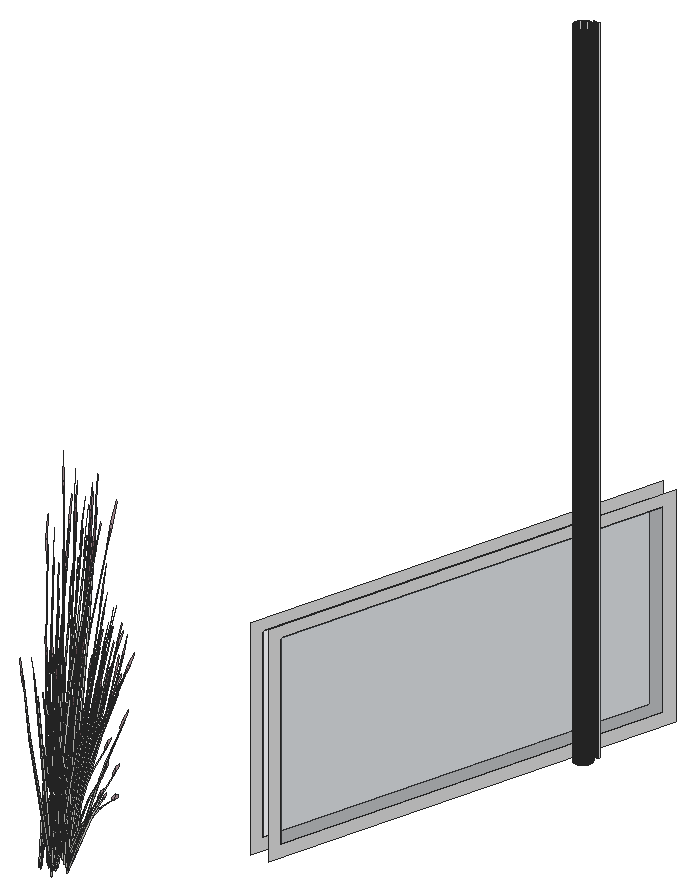
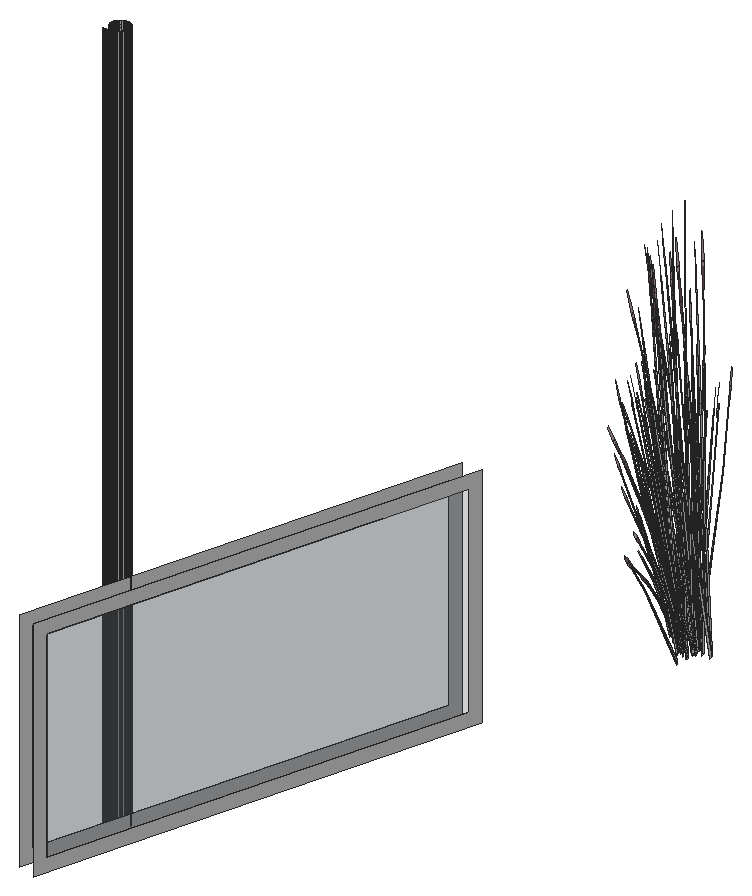
# SketchUp Ruby script. Lengths in inches.
U = 1.inch
M = Sketchup.active_model
def pt(a) = Geom::Point3d.new(a.map { |v| v * U })
def face(e, loops, mat)
  f = e.add_face(loops[0].map { |a| pt(a) })
  loops[1..].each { |l| e.add_face(l.map { |a| pt(a) }).erase! }
  f.material = f.back_material = mat if mat
  f
end
# faces: each face lists its corners as indices into pts; further lists are holes
def faces(e, pts, list, mat = nil) = list.each { |f| face(e, (f[0].is_a?(Array) ? f : [f]).map { |l| l.map { |i| pts[i] } }, mat) }
# xy, xz, yz: faces in a plane at the given z, y or x. An outline is a flat list of corners, or four numbers for a rectangle; further outlines are holes
def ring(l) = l.size == 4 ? [[l[0], l[1]], [l[2], l[1]], [l[2], l[3]], [l[0], l[3]]] : l.each_slice(2).to_a
def flat(e, list, mat, &to3) = list.each { |f| face(e, (f[0].is_a?(Array) ? f : [f]).map { |l| ring(l).map { |u, v| to3.(u, v) } }, mat) }
def xy(e, z, list, mat = nil) = flat(e, list, mat) { |x, y| [x, y, z] }
def xz(e, y, list, mat = nil) = flat(e, list, mat) { |x, z| [x, y, z] }
def yz(e, x, list, mat = nil) = flat(e, list, mat) { |y, z| [x, y, z] }
def lines(e, pts, list) = list.each { |a, b| e.add_line(pt(pts[a]), pt(pts[b])) }
# prism: a flat outline (further loops are holes) pulled along v
def prism(e, loops, v, mat = nil)
  f = face(e, loops, mat); d = Geom::Vector3d.new(v.map { |x| x * U })
  f.pushpull(f.normal.samedirection?(d) ? d.length : -d.length)
end
def box(e, o, s, mat = nil) = prism(e, [[o, [o[0] + s[0], o[1], o[2]], [o[0] + s[0], o[1] + s[1], o[2]], [o[0], o[1] + s[1], o[2]]]], [0, 0, s[2]], mat)
def at(x, y, z, deg = 0) = Geom::Transformation.translation(pt([x, y, z])) * Geom::Transformation.rotation(ORIGIN, Z_AXIS, deg.degrees)
def axes(o, x, y, z) = Geom::Transformation.new([*x, 0, *y, 0, *z, 0, *pt(o).to_a, 1])
def part(name) = M.definitions.add(name)
# library, detail: a bought-in or finely detailed component or shape, given as its bounding box
def library(name, o, s) = part(name).tap { |d| box(d.entities, o, s) }
def detail(e, o, s) = box(e.add_group.entities, o, s)
def put(e, d, t, mat = nil) = e.add_instance(d, t).tap { |i| i.material = mat if mat }
def group(e, t, mat = nil) = e.add_group.tap { |g| g.transformation = t; g.material = mat if mat }.entities
root = M.entities
M.materials.add("Glass_Basic_01").color = [105, 113, 122]
M.materials["Glass_Basic_01"].alpha = 0.25
M.materials.add("LightPink_Translucent").color = [144, 107, 117]
M.materials["LightPink_Translucent"].alpha = 0.75
M.materials.add("M01_Silver_Fog").color = [224, 224, 224]
c1 = part("blade")
p = [[2.15,0.21,22],[0,0.17,0],[0.09,0.45,0],[2.18,0.31,22],[2.29,0.31,22],[0.38,0.45,0],
  [2.48,0.24,33],[2.49,0.24,33],[2.48,0.22,33]]
faces(c1.entities,p,[[0,1,2,3],[4,5,2,3],[6,3,4,7],[8,0,3,6]])
c2 = part("seeds")
p = [[0.3,-0.1,1.38],[-0.01,-0.03,1.59],[-0.01,-0.03,0.03],[0.14,-0.07,-0.07],[0.29,-0.03,3],[0.15,0.01,3.11]]
faces(c2.entities,p,[[0,1,2,3],[1,0,4,5]],"LightPink_Translucent")
c3 = part("blade with seeds")
put(c3.entities,c1,at(0,0,0))
put(c3.entities,c2,axes([2.4,0.25,30.99],[1.5799,-0.05474,1.17369],[-0.12525,1.92788,0.29478],[-0.07173,-0.02425,1.56792]))
xz(root,421.6,[[358.82,270,358.91,384],[358.91,270,359,384]],"M01_Silver_Fog")
xz(root,421.95,[[359.74,270,359.83,384],[359.83,270,359.92,384]],"M01_Silver_Fog")
yz(root,357.51,[[420.11,270,420.2,384],[420.2,270,420.29,384]],"M01_Silver_Fog")
yz(root,360.31,[[420.11,270,420.2,384],[420.2,270,420.29,384]],"M01_Silver_Fog")
p = [[359.17,437.01,270],[340.07,371.78,270],[340.07,371.78,306],[359.17,437.01,306],[340.64,373.7,272],[358.6,435.09,272],
  [358.6,435.09,304],[340.64,373.7,304],[362.06,436.22,306],[343.2,371.78,306],[343.2,371.78,270],[362.06,436.22,270],
  [343.76,373.7,304],[361.5,434.3,304],[361.5,434.3,272],[343.76,373.7,272],[358.48,418.87,270],[358.5625,418.85,270],
  [358.5625,418.85,384],[358.48,418.87,384],[358.65,418.83,270],[358.73,418.8125,270],[358.73,418.8125,384],[358.65,418.83,384],
  [358.82,418.81,270],[358.82,418.81,384],[358.91,418.8,270],[358.91,418.8,384],[359,418.81,270],[359,418.81,384],
  [359.09,418.8125,270],[359.09,418.8125,384],[359.17,418.83,270],[359.17,418.83,384],[359.26,418.85,270],[359.26,418.85,384],
  [359.34,418.87,270],[359.34,418.87,384],[358.24,418.98,270],[358.3125,418.9375,270],[358.3125,418.9375,384],[358.24,418.98,384],
  [358.39,418.9,270],[358.39,418.9,384],[359.43,418.9,270],[359.43,418.9,384],[359.51,418.9375,270],[359.51,418.9375,384],
  [359.58,418.98,270],[359.58,418.98,384],[358.09,419.07,270],[358.16,419.02,270],[358.16,419.02,384],[358.09,419.07,384],
  [359.66,419.02,270],[359.66,419.02,384],[359.73,419.07,270],[359.73,419.07,384],[358.02,419.125,270],[358.02,419.125,384],
  [357.95,419.18,270],[357.95,419.18,384],[359.8,419.125,270],[359.8,419.125,384],[359.87,419.18,270],[359.87,419.18,384],
  [357.83,419.31,270],[357.89,419.24,270],[357.89,419.24,384],[357.83,419.31,384],[359.93,419.24,270],[359.93,419.24,384],
  [359.99,419.31,270],[359.99,419.31,384],[357.78,419.38,270],[357.78,419.38,384],[360.04,419.38,270],[360.04,419.38,384],
  [357.73,419.45,270],[357.73,419.45,384],[360.09,419.45,270],[360.09,419.45,384],[357.64,419.61,270],[357.68,419.53,270],
  [357.68,419.53,384],[357.64,419.61,384],[360.14,419.53,270],[360.14,419.53,384],[360.18,419.61,270],[360.18,419.61,384],
  [357.61,419.6875,270],[357.61,419.6875,384],[360.21,419.6875,270],[360.21,419.6875,384],[357.58,419.77,270],[357.58,419.77,384],
  [360.24,419.77,270],[360.24,419.77,384],[357.55,419.85,270],[357.55,419.85,384],[360.27,419.85,270],[360.27,419.85,384],
  [357.54,419.94,270],[357.54,419.94,384],[357.52,420.03,270],[357.52,420.03,384],[360.29,419.94,270],[360.29,419.94,384],
  [360.3,420.03,270],[360.3,420.03,384],[357.51,420.11,270],[357.51,420.11,384],[360.31,420.11,270],[360.31,420.11,384],
  [357.52,420.38,270],[357.51,420.29,270],[357.51,420.29,384],[357.52,420.38,384],[360.31,420.29,270],[360.3,420.38,270],
  [360.3,420.38,384],[360.31,420.29,384],[357.54,420.46,270],[357.54,420.46,384],[360.29,420.46,270],[360.29,420.46,384],
  [357.55,420.55,270],[357.55,420.55,384],[360.27,420.55,270],[360.27,420.55,384],[357.58,420.64,270],[357.58,420.64,384],
  [357.61,420.72,270],[357.61,420.72,384],[360.24,420.64,270],[360.24,420.64,384],[360.21,420.72,270],[360.21,420.72,384],
  [357.64,420.8,270],[357.64,420.8,384],[360.18,420.8,270],[360.18,420.8,384],[357.68,420.88,270],[357.68,420.88,384],
  [360.14,420.88,270],[360.14,420.88,384],[357.73,420.95,270],[357.73,420.95,384],[360.09,420.95,270],[360.09,420.95,384],
  [357.78,421.03,270],[357.78,421.03,384],[357.83,421.09,270],[357.83,421.09,384],[360.04,421.03,270],[360.04,421.03,384],
  [359.99,421.09,270],[359.99,421.09,384],[357.89,421.16,270],[357.89,421.16,384],[359.93,421.16,270],[359.93,421.16,384],
  [357.95,421.22,270],[357.95,421.22,384],[358.02,421.28,270],[358.02,421.28,384],[359.87,421.22,270],[359.8,421.28,270],
  [359.8,421.28,384],[359.87,421.22,384],[358.09,421.34,270],[358.09,421.34,384],[358.16,421.38,270],[358.16,421.38,384],
  [359.73,421.34,270],[359.73,421.34,384],[359.66,421.38,270],[359.66,421.38,384],[358.24,421.43,270],[358.24,421.43,384],
  [358.3125,421.47,270],[358.3125,421.47,384],[359.58,421.43,270],[359.51,421.47,270],[359.51,421.47,384],[359.58,421.43,384],
  [358.39,421.5,270],[358.39,421.5,384],[358.48,421.53,270],[358.48,421.53,384],[358.5625,421.56,270],[358.5625,421.56,384],
  [359.43,421.5,270],[359.34,421.53,270],[359.34,421.53,384],[359.43,421.5,384],[359.26,421.56,270],[359.26,421.56,384],
  [358.65,421.58,270],[358.65,421.58,384],[358.73,421.59,270],[358.73,421.59,384],[358.82,421.6,270],[358.82,421.6,384],
  [359.09,421.59,270],[359,421.6,270],[359,421.6,384],[359.09,421.59,384],[359.17,421.58,270],[359.17,421.58,384],
  [359.66,421.96,270],[359.74,421.95,270],[359.74,421.95,384],[359.66,421.96,384],[359.92,421.95,270],[360.01,421.96,270],
  [360.01,421.96,384],[359.92,421.95,384],[359.32,422.05,270],[359.4,422.02,270],[359.4,422.02,384],[359.32,422.05,384],
  [359.48,421.99,270],[359.48,421.99,384],[359.57,421.97,270],[359.57,421.97,384],[360.09,421.97,270],[360.09,421.97,384],
  [360.18,421.99,270],[360.18,421.99,384],[360.26,422.02,270],[360.26,422.02,384]]
faces(root,p,[[[0,1,2,3],[4,5,6,7]],[[8,9,10,11],[12,13,14,15]],[16,17,18,19],[20,21,22,23],[17,20,23,18],[21,24,25,22],[24,26,27,25],[26,28,29,27],
  [28,30,31,29],[30,32,33,31],[32,34,35,33],[34,36,37,35],[38,39,40,41],[39,42,43,40],[42,16,19,43],[36,44,45,37],
  [44,46,47,45],[46,48,49,47],[50,51,52,53],[51,38,41,52],[48,54,55,49],[54,56,57,55],[58,50,53,59],[60,58,59,61],
  [56,62,63,57],[62,64,65,63],[66,67,68,69],[67,60,61,68],[64,70,71,65],[70,72,73,71],[74,66,69,75],[72,76,77,73],
  [78,74,75,79],[76,80,81,77],[82,83,84,85],[83,78,79,84],[80,86,87,81],[86,88,89,87],[90,82,85,91],[88,92,93,89],
  [94,90,91,95],[92,96,97,93],[98,94,95,99],[96,100,101,97],[102,98,99,103],[104,102,103,105],[100,106,107,101],[106,108,109,107],
  [110,104,105,111],[108,112,113,109],[114,115,116,117],[118,119,120,121],[122,114,117,123],[119,124,125,120],[126,122,123,127],[124,128,129,125],
  [130,126,127,131],[132,130,131,133],[128,134,135,129],[134,136,137,135],[138,132,133,139],[136,140,141,137],[142,138,139,143],[140,144,145,141],
  [146,142,143,147],[144,148,149,145],[150,146,147,151],[152,150,151,153],[148,154,155,149],[154,156,157,155],[158,152,153,159],[156,160,161,157],
  [162,158,159,163],[164,162,163,165],[166,167,168,169],[160,166,169,161],[170,164,165,171],[172,170,171,173],[167,174,175,168],[174,176,177,175],
  [178,172,173,179],[180,178,179,181],[182,183,184,185],[176,182,185,177],[186,180,181,187],[188,186,187,189],[190,188,189,191],[192,193,194,195],
  [193,196,197,194],[183,192,195,184],[198,190,191,199],[200,198,199,201],[202,200,201,203],[204,205,206,207],[208,204,207,209],[196,208,209,197],
  [210,211,212,213],[214,215,216,217],[218,219,220,221],[219,222,223,220],[222,224,225,223],[224,210,213,225],[215,226,227,216],[226,228,229,227],
  [228,230,231,229]],"M01_Silver_Fog")
faces(root,p,[[5,4,7,6],[13,12,15,14]],"Glass_Basic_01")
put(root,c3,axes([325.91,345.85,276.68],[-0.35968,-0.36185,-0.51099],[0.37996,-0.3169,-0.3958],[0.05473,-0.18385,0.97773]))
put(root,c3,axes([326.25,345.72,276.53],[0.33997,-0.28354,-0.35414],[0.32182,0.32376,0.4572],[0.04897,-0.1645,0.87481]))
put(root,c3,axes([326.68,345.55,273.49],[-0.0752,-0.04243,1.76342],[-0.19317,-0.47398,-0.26939],[0.13031,-0.12863,0.30037]))
put(root,c3,axes([326.25,345.83,276.73],[0.35779,0.36745,0.48003],[-0.37996,0.3169,0.3958],[0.066,-0.17239,0.9933]))
put(root,c3,axes([326.38,345.86,276.73],[0.4129,0.02509,0.0643],[-0.01132,0.37891,0.50621],[0.04321,-0.14514,0.77189]))
put(root,c3,axes([326.08,346.12,277.05],[-0.33997,0.28354,0.35414],[-0.32182,-0.32376,-0.4572],[0.04897,-0.1645,0.87481]))
put(root,c3,axes([326.67,346.88,276.98],[0.26246,-0.42493,-0.71045],[0.45991,0.30199,0.08574],[0.15671,-0.15395,1.00501]))
put(root,c3,axes([326.66,346.68,276.68],[-0.12908,-0.49174,-0.51099],[0.48882,-0.08602,-0.3958],[0.14008,-0.13208,0.97773]))
put(root,c3,axes([326.89,347.04,277.03],[-0.46478,-0.29695,-0.1216],[0.26776,-0.43004,-0.67495],[0.13131,-0.14949,1.02557]))
put(root,c3,axes([324.26,345.5625,274.02],[0.47024,-0.26927,-0.49651],[0.28107,0.48284,0],[0.1071,-0.06133,1.57504]))
put(root,c3,axes([327.05,346.49,274.59],[-0.1795,-0.01595,1.43002],[-0.18389,-0.42791,-0.30754],[0.22051,-0.12105,0.61141]))
put(root,c3,axes([328.04,346.91,276.71],[-0.06563,-0.00409,1.77383],[-0.27252,-0.43825,-0.16761],[0.10944,-0.1441,0.31391]))
put(root,c3,axes([324.82,346.67,274.06],[0.33843,-0.40479,-0.62353],[0.42041,0.36705,-0.16365],[0.13561,-0.10098,1.37633]))
put(root,c3,axes([327.26,345.71,274.77],[-0.16736,0.27414,1.1486],[-0.14385,-0.36832,0.84392],[0.13822,-0.09229,0.25299]))
put(root,c3,axes([327.02,346.74,276.53],[0.43736,-0.07697,-0.35414],[0.11549,0.43998,0.4572],[0.12533,-0.11818,0.87481]))
put(root,c3,axes([324.45,347.14,274.67],[-0.05855,-0.61451,-0.29095],[0.60981,-0.03716,-0.50002],[0.10738,-0.08185,1.59708]))
put(root,c3,axes([326.67,347,277.05],[-0.43736,0.07697,0.35414],[-0.11549,-0.43998,-0.4572],[0.12533,-0.11818,0.87481]))
put(root,c3,axes([324.375,345.77,274.03],[0.46876,0.13325,-0.30978],[-0.11803,0.46926,0.30978],[0.0945,-0.05411,1.38974]))
put(root,c3,axes([327.0625,346.93,276.73],[0.34493,0.22649,0.0643],[-0.20082,0.32253,0.50621],[0.11059,-0.10427,0.77189]))
put(root,c3,axes([326.97,346.83,276.73],[0.12461,0.49565,0.48003],[-0.48882,0.08602,0.3958],[0.14406,-0.11657,0.9933]))
put(root,c3,axes([328.28,347.43,276.72],[0.06972,-0.08203,1.74944],[-0.08924,-0.50318,-0.27667],[0.17494,-0.0954,0.14031]))
put(root,c3,axes([326.91,348.19,277.03],[-0.25281,-0.48765,-0.1216],[0.44869,-0.23964,-0.67495],[0.18908,-0.06434,1.02557]))
put(root,c3,axes([326.89,347.78,276.68],[0.13612,-0.48987,-0.51099],[0.46669,0.16791,-0.3958],[0.1879,-0.04492,0.97773]))
put(root,c3,axes([326.15,345.78,274.375],[0.31414,-0.53965,0],[0.52557,0.30095,-0.51607],[0.1197,0.06854,1.63711]))
put(root,c3,axes([327.39,347.91,273.98],[-0.32361,0.06463,1.41583],[-0.05151,-0.51444,0.08104],[0.22666,-0.07786,0.80566]))
put(root,c3,axes([327.98,347.46,274.26],[-0.31151,-0.34437,-0.06488],[0.34117,-0.31553,-0.29416],[0.09667,-0.02221,0.97024]))
put(root,c3,axes([325.88,346.0625,274.48],[-0.47024,-0.26927,0.49651],[0.28107,-0.48284,0],[0.1071,0.06133,1.57504]))
put(root,c3,axes([326.8,347.95,276.98],[0.44151,-0.23785,-0.71045],[0.24605,0.4896,0.08574],[0.21333,-0.05562,1.00501]))
put(root,c3,axes([326.74,348.05,277.05],[-0.41757,-0.15024,0.35414],[0.12179,-0.4383,-0.4572],[0.16812,-0.04019,0.87481]))
put(root,c3,axes([323.88,346.74,273.59],[-0.49456,0.21561,1.28929],[-0.15741,-0.61865,0.50096],[0.30369,0.01029,1.46642]))
put(root,c3,axes([325.21,346.9,274.62],[0.09693,-0.48062,0.1448],[0.47357,0.08343,-0.41347],[0.08619,0.04935,1.26744]))
put(root,c3,axes([327.74,347.58,273.49],[-0.02626,-0.08176,1.76342],[0.18213,-0.47826,-0.26939],[0.18372,-0.00688,0.30037]))
put(root,c3,axes([325,347.03,274.72],[-0.30184,-0.45202,0.44739],[0.45719,-0.31831,-0.21531],[0.09768,0.05593,1.43643]))
put(root,c3,axes([325.16,347.06,274.67],[0.5073,-0.35754,-0.29095],[0.33735,0.5052,-0.50002],[0.12516,0.05131,1.59708]))
put(root,c3,axes([327.18,348,276.53],[0.41757,0.15024,-0.35414],[-0.12179,0.4383,0.4572],[0.16812,-0.04019,0.87481]))
put(root,c3,axes([326.4375,346.11,274.02],[0.47024,0.26927,-0.49651],[-0.28107,0.48284,0],[0.1071,0.06133,1.57504]))
put(root,c3,axes([325.54,347.64,274.21],[0.56215,0,0],[0,0.55754,0],[0,0,1.78407]))
put(root,c3,axes([326.04,347.46,275.875],[-0.20841,0.0122,1.71376],[0.13825,-0.52864,0.13857],[0.297,0.0327,0.73262]))
put(root,c3,axes([326.31,346.31,274.03],[0.11803,0.46926,-0.30978],[-0.46876,0.13325,0.30978],[0.0945,0.05411,1.38974]))
put(root,c3,axes([327.11,348.18,276.73],[0.18454,0.3672,0.0643],[-0.33652,0.17973,0.50621],[0.14834,-0.03546,0.77189]))
put(root,c3,axes([327.08,348.05,276.73],[-0.14195,0.49104,0.48003],[-0.46669,-0.16791,0.3958],[0.18353,-0.02951,0.9933]))
put(root,c3,axes([325.47,348.875,274.18],[0.5275,-0.18273,-0.19198],[0.18536,0.52636,0.00008],[0.05823,-0.0202,1.73897]))
put(root,c3,axes([325.75,347.14,274.06],[0.52267,0.08829,-0.62353],[-0.11029,0.54463,-0.16365],[0.15598,0.06599,1.37633]))
put(root,c3,axes([328.0625,348.09,274.77],[-0.31044,0.08891,1.1486],[0.14613,-0.36744,0.84392],[0.16469,0.02514,0.25299]))
put(root,c3,axes([327.92,349.64,276.71],[-0.04543,-0.04715,1.77383],[0.09938,-0.50538,-0.16761],[0.17896,-0.03229,0.31391]))
put(root,c3,axes([325.48,347.3125,274.21],[0.30184,0.45202,-0.44739],[-0.45719,0.31831,0.21531],[0.09768,0.05593,1.43643]))
put(root,c3,axes([327.52,349.22,275.93],[-0.09617,-0.45271,-0.03492],[0.45453,-0.10408,-0.15832],[0.09492,0.0287,0.52218]))
put(root,c3,axes([326.34,349.21,277.03],[0.0269,-0.54769,-0.1216],[0.50939,0.01497,-0.67495],[0.19618,0.03804,1.02557]))
put(root,c3,axes([326.81,347.74,274.48],[0,-0.53854,0.49651],[0.56215,0,0],[0,0.12266,1.57504]))
put(root,c3,axes([325.74,347.59,274.62],[0.46814,-0.15705,0.1448],[0.16394,0.44848,-0.41347],[0,0.0987,1.26744]))
put(root,c3,axes([326.27,348.99,277.05],[-0.28589,-0.33718,0.35414],[0.32644,-0.31919,-0.4572],[0.16586,0.04856,0.87481]))
put(root,c3,axes([327.48,348.68,274.59],[-0.12101,-0.13245,1.43002],[0.15744,-0.43816,-0.30754],[0.24483,0.05936,0.61141]))
put(root,c3,axes([326.79,348.88,276.72],[0.10779,-0.00911,1.74944],[0.29564,-0.41839,-0.27667],[0.19172,0.05523,0.14031]))
put(root,c3,axes([326.37,348.94,276.98],[0.50227,0.01297,-0.71045],[-0.03373,0.54602,0.08574],[0.21278,0.05762,1.00501]))
put(root,c3,axes([327.1875,347.84,274.375],[0.62828,0,0],[0,0.6019,-0.51607],[0,0.13709,1.63711]))
put(root,c3,axes([325.58,347.62,274.67],[0.56585,0.25696,-0.29095],[-0.27246,0.54236,-0.50002],[0.01778,0.13316,1.59708]))
put(root,c3,axes([326.67,349.17,276.53],[0.28589,0.33718,-0.35414],[-0.32644,0.31919,0.4572],[0.16586,0.04856,0.87481]))
put(root,c3,axes([326.52,349.3,276.73],[-0.0253,0.40952,0.0643],[-0.38204,-0.01123,0.50621],[0.14634,0.04285,0.77189]))
put(root,c3,axes([326.56,349.17,276.73],[-0.37048,0.35486,0.48003],[-0.31952,-0.37685,0.3958],[0.17382,0.06546,0.9933]))
put(root,c3,axes([325.38,349.58,277.05],[-0.0776,-0.43378,0.35414],[0.44361,-0.11454,-0.4572],[0.11915,0.12431,0.87481]))
put(root,c3,axes([327.05,348.25,274.02],[0,0.53854,-0.49651],[-0.56215,0,0],[0,0.12266,1.57504]))
put(root,c3,axes([325.64,348.31,275.875],[-0.18664,-0.09279,1.71376],[0.38624,-0.38925,0.13857],[0.24072,0.1756,0.73262]))
put(root,c3,axes([325.68,347.08,276.47],[-0.43417,-0.27982,1.38283],[0.45844,-0.43566,0.59665],[0.14008,0.26255,1.33663]))
put(root,c3,axes([326.33,349.36,274.77],[-0.2829,-0.15485,1.1486],[0.36529,-0.15734,0.84392],[0.09853,0.13328,0.25299]))
put(root,c3,axes([325.34,349.8,277.03],[0.2994,-0.46097,-0.1216],[0.43359,0.26557,-0.67495],[0.15072,0.13024,1.02557]))
put(root,c3,axes([324.95,350.1875,276.71],[0.00149,-0.0652,1.77383],[0.43058,-0.28766,-0.16761],[0.14956,0.10267,0.31391]))
put(root,c3,axes([326.41,349.9375,273.49],[0.03661,-0.07775,1.76342],[0.46087,-0.22898,-0.26939],[0.13972,0.11851,0.30037]))
put(root,c3,axes([325.7,349.58,276.68],[0.4958,-0.12802,-0.51099],[0.08673,0.48481,-0.3958],[0.13317,0.13893,0.97773]))
put(root,c3,axes([326.38,350.07,274.67],[-0.3222,-0.01689,1.0506],[0.21278,-0.35872,0.58006],[0.12729,0.12745,0.8241]))
put(root,c3,axes([325.45,349.97,276.73],[-0.22836,0.34211,0.0643],[-0.3252,-0.19918,0.50621],[0.10513,0.10968,0.77189]))
put(root,c3,axes([325.55,349.875,276.73],[-0.49974,0.12359,0.48003],[-0.08673,-0.48481,0.3958],[0.11753,0.14288,0.9933]))
put(root,c3,axes([325.33,349.2,274.59],[0.00887,-0.17852,1.43002],[0.42372,-0.19941,-0.30754],[0.1308,0.21367,0.61141]))
put(root,c3,axes([324.875,348.84,275.875],[-0.11485,-0.17291,1.71376],[0.53072,-0.14557,0.13857],[0.11995,0.27145,0.73262]))
